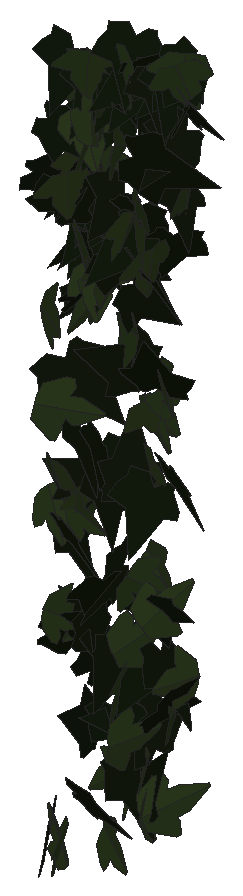
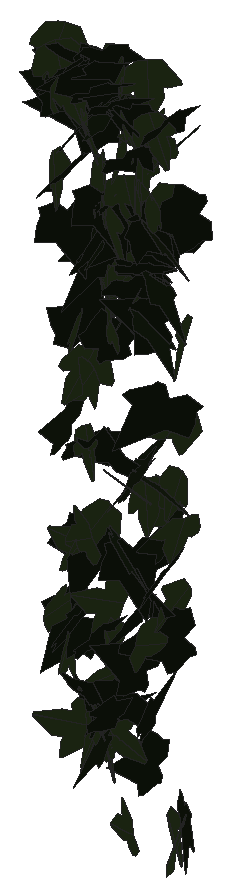
# SketchUp Ruby script. Lengths in inches.
U = 1.inch
M = Sketchup.active_model
def pt(a) = Geom::Point3d.new(a.map { |v| v * U })
def face(e, loops, mat)
  f = e.add_face(loops[0].map { |a| pt(a) })
  loops[1..].each { |l| e.add_face(l.map { |a| pt(a) }).erase! }
  f.material = f.back_material = mat if mat
  f
end
# faces: each face lists its corners as indices into pts; further lists are holes
def faces(e, pts, list, mat = nil) = list.each { |f| face(e, (f[0].is_a?(Array) ? f : [f]).map { |l| l.map { |i| pts[i] } }, mat) }
# xy, xz, yz: faces in a plane at the given z, y or x. An outline is a flat list of corners, or four numbers for a rectangle; further outlines are holes
def ring(l) = l.size == 4 ? [[l[0], l[1]], [l[2], l[1]], [l[2], l[3]], [l[0], l[3]]] : l.each_slice(2).to_a
def flat(e, list, mat, &to3) = list.each { |f| face(e, (f[0].is_a?(Array) ? f : [f]).map { |l| ring(l).map { |u, v| to3.(u, v) } }, mat) }
def xy(e, z, list, mat = nil) = flat(e, list, mat) { |x, y| [x, y, z] }
def xz(e, y, list, mat = nil) = flat(e, list, mat) { |x, z| [x, y, z] }
def yz(e, x, list, mat = nil) = flat(e, list, mat) { |y, z| [x, y, z] }
def lines(e, pts, list) = list.each { |a, b| e.add_line(pt(pts[a]), pt(pts[b])) }
# prism: a flat outline (further loops are holes) pulled along v
def prism(e, loops, v, mat = nil)
  f = face(e, loops, mat); d = Geom::Vector3d.new(v.map { |x| x * U })
  f.pushpull(f.normal.samedirection?(d) ? d.length : -d.length)
end
def box(e, o, s, mat = nil) = prism(e, [[o, [o[0] + s[0], o[1], o[2]], [o[0] + s[0], o[1] + s[1], o[2]], [o[0], o[1] + s[1], o[2]]]], [0, 0, s[2]], mat)
def at(x, y, z, deg = 0) = Geom::Transformation.translation(pt([x, y, z])) * Geom::Transformation.rotation(ORIGIN, Z_AXIS, deg.degrees)
def axes(o, x, y, z) = Geom::Transformation.new([*x, 0, *y, 0, *z, 0, *pt(o).to_a, 1])
def part(name) = M.definitions.add(name)
# library, detail: a bought-in or finely detailed component or shape, given as its bounding box
def library(name, o, s) = part(name).tap { |d| box(d.entities, o, s) }
def detail(e, o, s) = box(e.add_group.entities, o, s)
def put(e, d, t, mat = nil) = e.add_instance(d, t).tap { |i| i.material = mat if mat }
def group(e, t, mat = nil) = e.add_group.tap { |g| g.transformation = t; g.material = mat if mat }.entities
root = M.entities
M.materials.add("efeu1").color = [18, 25, 13]
M.materials.add("efeu2").color = [43, 57, 29]
c1 = part("ivyleaf_9")
p = [[1.54,2.16,1.25],[1.36,2.04,1.19],[-0.21,0.99,0.68],[-0.71,1.11,0.82],[-0.85,0.86,0.67],[-0.8,0.17,0.21],
  [-0.9,-0.01,0.1],[-0.67,-0.16,-0.02],[-0.08,-0.08,-0.05],[-0.03,-0.6,-0.4],[0.65,-0.88,-0.66],[0.83,-0.6,-0.49],
  [1.29,-0.42,-0.43],[1.8125,-0.07,-0.26],[1.21,0.44,0.15]]
faces(c1.entities,p,[[0,1,2,3,4,5,6,7,8,9,10,11,12,13,14]],"efeu1")
c2 = part("ivyleaf_10")
p = [[0,0.5,-0.03],[-0.0625,2.02,-0.43],[-0.19,2.01,-0.46],[-0.54,1.05,-0.29],[-0.52,0.625,-0.18],[-0.83,0.76,-0.28],
  [-1.16,0.64,-0.33],[-1.15,0.33,-0.24],[-0.77,-0.39,0.02],[-0.3,-0.51,0.16],[0.04,-0.48,0.23],[-0.02,2.01,-0.4375],
  [-0.06,2.01,-0.43],[0.04,-0.49,0.23],[0.67,-0.49,0.14],[1.38,0.36,-0.2],[1.375,0.51,-0.24],[0.81,0.65,-0.19],
  [0.62,0.59,-0.15],[0.6,1.09,-0.28],[0.5,1.23,-0.31]]
faces(c2.entities,p,[[0,1,2,3,4,5,6,7,8,9,10],[11,12,0,13,14,15,16,17,18,19,20]],"efeu2")
put(root,c1,axes([558.99,128.62,206.93],[-0.14033,0.02184,-1.08873],[-1.0012,0.42913,0.13765],[0.42827,1.01038,-0.03493]))
put(root,c2,axes([558.67,129.81,205.36],[-0.53555,0.90235,-0.1716],[-0.12374,0.12595,1.04848],[0.91014,0.54809,0.04157]))
put(root,c2,axes([558.25,129.72,221.42],[0.26299,0.95751,0.15924],[0.04787,0.15199,-0.99295],[-0.96948,0.26725,-0.00583]))
put(root,c2,axes([558.71,128.875,230.33],[-0.41315,0.69461,0.69183],[-0.42365,0.55054,-0.80575],[-0.8841,-0.58841,0.06281]))
put(root,c1,axes([557.92,129.1875,236.32],[0.17224,0.54015,-0.81604],[0.28185,0.76609,0.56658],[0.93715,-0.32968,-0.02042]))
put(root,c1,axes([558.34,130.9375,241.17],[-0.27235,-0.93235,0.29323],[-0.01478,-0.30044,-0.96899],[0.97726,-0.26437,0.06706]))
put(root,c1,axes([559.01,130.45,233.21],[-0.61672,0.77611,-0.04246],[0.03203,-0.02879,-0.99128],[-0.77661,-0.61751,-0.00716]))
put(root,c1,axes([558.23,130.81,219.78],[0.48249,-0.80704,-0.27],[-0.14212,0.2296,-0.94027],[0.83906,0.50297,-0.00401]))
put(root,c1,axes([559.04,130.875,235.99],[-0.8604,0.40877,-0.20405],[0.16752,-0.12253,-0.95181],[-0.42505,-0.87574,0.03792]))
put(root,c2,axes([559.12,130.72,240.85],[-0.85129,-0.027,0.49047],[-0.47595,-0.19735,-0.83696],[0.12148,-0.96245,0.15786]))
put(root,c1,axes([559.45,130.33,230.87],[-0.35302,0.84005,0.36834],[-0.31546,0.25941,-0.89396],[-0.8613,-0.43932,0.17645]))
put(root,c2,axes([558.89,129.25,223.13],[-0.86155,0.40048,-0.04378],[0.0411,-0.01544,-0.95007],[-0.40077,-0.86252,-0.00332]))
put(root,c2,axes([559.09,130.33,236.95],[0.01574,-0.90176,0.44705],[0.02742,-0.44655,-0.90173],[1.00612,0.02628,0.01758]))
put(root,c1,axes([559.12,131.28,236.4375],[-0.30759,0.37254,-0.86401],[0.44342,-0.74434,-0.4788],[-0.82987,-0.53581,0.06441]))
put(root,c2,axes([559.0625,129.375,206.56],[0.48481,-0.8241,0.02003],[0.01483,-0.01451,-0.95611],[0.82421,0.485,0.00543]))
put(root,c1,axes([559.8,129.625,222.84],[-0.36512,0.6723,0.51093],[-0.54966,0.23334,-0.69984],[-0.64102,-0.58302,0.30907]))
put(root,c1,axes([558.51,129.7,234.65],[-0.08443,-0.16044,0.99072],[1.00342,0.00694,0.08663],[-0.02063,0.99429,0.15926]))
put(root,c2,axes([559.21,131.25,216.0625],[0.0966,0.37472,-0.88999],[-0.25262,-0.85347,-0.38677],[-0.93203,0.27016,0.01259]))
put(root,c2,axes([559.29,129.4375,236.31],[-0.49063,-0.8754,-0.07136],[0.02747,0.0664,-1.00348],[0.87788,-0.49133,-0.00848]))
put(root,c1,axes([558.64,130.23,227.54],[-0.08979,-0.46984,-1.10499],[0.35695,1.04754,-0.47442],[1.14645,-0.36295,0.06117]))
put(root,c2,axes([558.62,129.08,226.04],[-0.13884,-0.24942,-1.05061],[0.96555,0.44555,-0.23337],[0.48342,-0.96153,0.16439]))
put(root,c2,axes([559.32,128.4375,217.12],[-0.04611,0.53566,0.801],[-0.13304,0.7907,-0.53643],[-0.95438,-0.13611,0.03608]))
put(root,c1,axes([558.7,129.22,215.64],[0.6801,0.26796,0.73486],[0.68349,0.26993,-0.73098],[-0.38035,0.96421,0.00042]))
put(root,c1,axes([559.4375,131.46,234.24],[-0.78252,-0.61482,0.02829],[0.13153,-0.21175,-0.96385],[0.60126,-0.75386,0.24766]))
put(root,c1,axes([559,128.67,239.25],[0.70392,-0.50862,-0.52755],[-0.16527,0.60247,-0.80138],[0.71392,0.64097,0.33463]))
put(root,c1,axes([559.65,131.09,234.16],[-0.79091,-0.55455,-0.11469],[0.09217,0.06832,-0.96595],[0.55873,-0.79626,-0.003]))
put(root,c1,axes([559.08,129.39,220.6],[0.6914,-0.5788,0.15277],[0.11818,-0.09683,-0.90169],[0.58684,0.70143,0.00159]))
put(root,c1,axes([559.45,130.46,233.45],[0.66187,-0.53962,-0.55674],[-0.40225,0.3868,-0.85311],[0.66284,0.77357,0.03821]))
put(root,c1,axes([559.34,129.76,230.8],[0.18284,0.92021,-0.39849],[0.0771,0.39095,0.9382],[0.99982,-0.19843,0.00052]))
put(root,c1,axes([559.89,130.1875,211.32],[-0.15828,0.0297,0.95286],[-0.32432,-0.90997,-0.02551],[0.89646,-0.32396,0.15901]))
put(root,c1,axes([559.4375,130.16,224.61],[0.3603,-0.90096,0.33872],[0.12813,-0.31356,-0.97033],[0.95396,0.3824,0.0024]))
put(root,c2,axes([559.66,130.98,237.56],[0.55503,-0.64106,0.48861],[0.48472,-0.20853,-0.8242],[0.644,0.70944,0.19925]))
put(root,c2,axes([560.16,129.75,222.45],[-0.21734,-0.92722,-0.07315],[0.01697,0.07115,-0.95235],[0.92994,-0.218,0.00029]))
put(root,c2,axes([560.17,129.84,238.41],[0.20873,-0.88624,-0.43695],[-0.01941,0.44282,-0.90744],[0.98791,0.19595,0.07449]))
put(root,c1,axes([560.08,131.25,239.17],[-0.53453,-0.8444,0.10638],[0.01515,-0.13504,-0.99579],[0.85094,-0.52802,0.08455]))
put(root,c1,axes([559.67,131.15,223.6],[0.08003,-0.70565,0.66439],[0.17582,-0.64502,-0.70626],[0.95312,0.17823,0.07449]))
put(root,c1,axes([559.99,131.03,233.08],[-0.4486,-0.83389,-0.21901],[0.16097,0.16153,-0.94476],[0.84701,-0.47235,0.06355]))
put(root,c1,axes([560.3,130.47,241],[-0.84195,-0.49876,-0.15488],[0.1388,0.06956,-0.97853],[0.50347,-0.85325,0.01076]))
put(root,c2,axes([560.45,129.35,242.29],[-0.78359,-0.66818,0.08016],[-0.06965,-0.04185,-1.02971],[0.66936,-0.78657,-0.01331]))
put(root,c2,axes([560.57,130.64,237.3125],[-0.9298,-0.1154,0.30767],[-0.27239,-0.24579,-0.91537],[0.1838,-0.94804,0.19987]))
put(root,c2,axes([560.21,130.14,231.15],[-0.0111,-0.40165,0.90513],[0.21172,-0.88521,-0.39022],[0.96734,0.18913,0.09579]))
put(root,c1,axes([561,128.95,216.64],[-0.25972,0.29871,0.94969],[-0.61467,0.72396,-0.39581],[-0.78315,-0.66727,-0.0043]))
put(root,c2,axes([560.19,129.03,234.25],[-0.68525,0.6821,-0.13138],[0.08987,-0.09595,-0.96685],[-0.6888,-0.6911,0.00456]))
put(root,c1,axes([560.36,131.3,223.51],[-0.8108,-0.24209,-0.34921],[0.40316,-0.20065,-0.79697],[0.13422,-0.8597,0.28434]))
put(root,c2,axes([560.52,129.26,239.06],[-0.09308,0.93086,-0.54961],[-0.1256,0.5386,0.93348],[1.07369,0.1437,0.06155]))
put(root,c1,axes([559.98,130.14,214.08],[0.13359,-0.11991,1.05032],[0.78522,0.72009,-0.01766],[-0.70781,0.77621,0.17864]))
put(root,c1,axes([560.91,130.75,240.5],[-0.97074,0.21539,0.07325],[-0.07451,0.00233,-0.99426],[-0.21496,-0.9735,0.01383]))
put(root,c2,axes([560,129.45,239.27],[0.7958,0.55612,0.33148],[0.2758,0.184,-0.97084],[-0.58573,0.84221,-0.00678]))
put(root,c2,axes([559.75,129.22,221.58],[0.07631,-0.1076,0.90905],[0.91477,0.04286,-0.07172],[-0.03402,0.91124,0.11071]))
put(root,c2,axes([560.35,129.73,232.33],[0.63947,0.7254,0.09194],[0.05587,0.07331,-0.96699],[-0.72906,0.64187,0.00654]))
put(root,c1,axes([560.23,129.01,208.86],[0.73504,-0.38675,0.48989],[0.44125,-0.21331,-0.83045],[0.44144,0.85719,0.01437]))
put(root,c2,axes([560.27,130.65,206.31],[0.27672,-0.04353,0.97521],[0.94609,-0.23776,-0.27907],[0.24049,0.98543,-0.02426]))
put(root,c2,axes([560.99,130.02,240.53],[0.37829,-0.89853,0.15926],[0.08484,-0.13702,-0.9746],[0.90858,0.3869,0.0247]))
put(root,c1,axes([561.27,129.21,218.86],[0.16936,0.88596,-0.48783],[-0.0822,-0.48093,-0.90196],[-1.00804,0.18806,-0.00841]))
put(root,c2,axes([561.19,129.99,232.85],[-0.1984,-0.95037,0.21572],[-0.02604,-0.21489,-0.97069],[0.9742,-0.19929,0.01799]))
put(root,c1,axes([560.66,130.15,222.73],[0.21157,-0.965,0.20893],[0.04249,-0.20457,-0.98792],[0.98644,0.21579,-0.00226]))
put(root,c1,axes([561.09,130.97,241.22],[-0.61139,-0.7967,0.11583],[0.11322,-0.22909,-0.97808],[0.79708,-0.57855,0.22778]))
put(root,c1,axes([561.45,131.3,211.76],[-0.05574,-0.69209,-0.58924],[-0.01887,-0.58934,0.69399],[-0.90875,0.05469,0.02173]))
put(root,c1,axes([561.7,129.79,219.45],[-0.92418,0.45294,-0.32855],[0.29713,-0.14028,-1.0292],[-0.47415,-0.97076,-0.00457]))
put(root,c2,axes([561.97,129.93,210.24],[-0.43773,-0.25611,0.80676],[-0.6712,-0.44833,-0.5065],[0.5157,-0.80091,0.02555]))
put(root,c2,axes([561.59,129.53,238.75],[0.25822,-0.48953,-0.86004],[-0.14162,0.86141,-0.53283],[0.97941,0.25362,0.1497]))
put(root,c1,axes([560.94,130.25,212.52],[-0.29374,-0.31991,-0.87643],[0.63983,0.59967,-0.43333],[0.67904,-0.70343,0.02918]))
put(root,c1,axes([561.24,129.99,215.45],[-0.0653,-0.97947,0.57005],[-0.04544,-0.56827,-0.98162],[1.13236,-0.07928,-0.00652]))
put(root,c1,axes([561.54,130.09,236.18],[-0.34519,-0.75817,0.56128],[-0.07354,-0.57423,-0.82089],[0.94045,-0.32319,0.14183]))
put(root,c2,axes([562.1,129.94,234.91],[0.66039,-0.42115,-0.66754],[-0.50251,0.44685,-0.77904],[0.60866,0.82587,0.0811]))
put(root,c1,axes([562.1,129.88,223.26],[-1.05025,0.14244,0.21134],[0.20818,-0.03756,1.05982],[0.14703,1.07064,0.00906]))
put(root,c2,axes([561.79,130,214.72],[0.52408,-1.03025,0.2683],[0.11556,-0.24223,-1.15587],[1.05832,0.53663,-0.00665]))
put(root,c2,axes([561.64,129.81,242.56],[-0.68138,0.48042,-0.54987],[0.33141,-0.46669,-0.81842],[-0.65063,-0.74084,0.15898]))
put(root,c1,axes([561.7,130.51,210.33],[0.78926,-0.39965,-0.35194],[-0.30862,0.16952,-0.88461],[0.43397,0.84738,0.01098]))
put(root,c1,axes([562.08,131,241.52],[-0.63703,-0.7684,0.18306],[0.03067,-0.25906,-0.98067],[0.78931,-0.61008,0.18585]))
put(root,c1,axes([562.375,129.86,235.9],[0.4044,0.54385,-0.7747],[-0.42202,-0.65047,-0.67694],[-0.84725,0.58359,-0.03258]))
put(root,c1,axes([562.49,129.83,228.67],[-0.04315,-0.05191,1.03692],[-0.90311,-0.51007,-0.06312],[0.51214,-0.90382,-0.02394]))
put(root,c1,axes([562.47,130.64,242.0625],[-0.77811,-0.5283,0.39865],[-0.32311,-0.23376,-0.94044],[0.5776,-0.84245,0.01096]))
put(root,c1,axes([561.94,130.4,243.27],[-0.54641,-0.77859,-0.31056],[0.2449,0.20626,-0.948],[0.80167,-0.59369,0.07792]))
put(root,c1,axes([561.5,130.54,240.37],[0.41774,-0.85171,0.28529],[0.31362,-0.15653,-0.92652],[0.84169,0.48103,0.20364]))
put(root,c2,axes([562.21,129.98,209.88],[0.58641,-0.77525,-0.09309],[-0.05635,0.07411,-0.97206],[0.77879,0.58911,-0.00023]))
put(root,c1,axes([561.89,128.97,234.13],[0.07976,-0.092,-1.02629],[-0.06477,1.02688,-0.09708],[1.02837,0.07181,0.07348]))
put(root,c2,axes([561.72,130.14,230.07],[0.56125,-0.3845,0.69192],[0.6574,-0.24606,-0.66998],[0.44093,0.85628,0.11817]))
put(root,c1,axes([562.29,130.75,214.96],[-0.29919,-0.83094,0.40734],[-0.11496,-0.39141,-0.88288],[0.91824,-0.31975,0.02219]))
put(root,c2,axes([563.02,128.8,230.99],[0.16737,-0.23559,-1.0808],[-0.69784,0.82565,-0.28804],[0.85829,0.71725,-0.02344]))
put(root,c1,axes([562.72,129.57,235],[-0.72792,-0.62121,0.29921],[-0.21163,-0.2128,-0.95667],[0.65623,-0.7577,0.02338]))
put(root,c2,axes([562.46,129.27,235.59],[0.15148,-0.92723,0.34655],[0.13361,-0.32822,-0.9366],[0.98081,0.18791,0.07406]))
put(root,c2,axes([562.17,129.37,216.21],[0.20845,0.31534,-0.9882],[0.6122,0.77628,0.37685],[0.83737,-0.64604,-0.02953]))
put(root,c2,axes([563.08,129.21,236.82],[-0.61335,0.39923,0.74009],[-0.67475,0.31301,-0.72805],[-0.50183,-0.90883,0.07436]))
put(root,c1,axes([563.14,130.14,211.68],[-1.06679,0.20701,-0.21356],[-0.21057,0.0359,1.08668],[0.21004,1.08736,0.00478]))
put(root,c2,axes([563.02,130.24,224.29],[-0.70586,0.30113,0.51014],[-0.5129,0.08637,-0.76067],[-0.29639,-0.86661,0.10145]))
put(root,c2,axes([562.49,130.82,239.59],[0.71658,-0.64273,0.24249],[0.16228,-0.18211,-0.96223],[0.66751,0.73425,-0.02639]))
put(root,c1,axes([562.14,130.04,241.74],[0.59621,0.23261,0.76126],[0.68152,0.34226,-0.63834],[-0.41128,0.90435,0.04578]))
put(root,c2,axes([562.54,128.53,212.33],[-0.04399,-0.05123,-1.07154],[0.46708,0.96454,-0.06528],[0.96575,-0.46883,-0.01723]))
put(root,c2,axes([562.9,129.67,210.95],[0.65049,-0.76511,-0.13929],[-0.08862,0.10748,-1.00426],[0.77262,0.6565,0.00208]))
put(root,c1,axes([562.4375,129.16,210.9],[0.41602,-0.94136,-0.35014],[-0.12257,0.32858,-1.029],[0.99686,0.43326,0.01961]))
put(root,c1,axes([562.83,129.29,232.84],[0.29116,-0.37408,-0.94032],[-0.39938,0.85657,-0.46442],[0.92986,0.48504,0.09496]))
put(root,c1,axes([562.58,131.05,239.79],[0.39403,-0.92841,-0.05768],[0.01367,0.06842,-1.0078],[0.9301,0.39231,0.03925]))
put(root,c2,axes([563.33,131.11,241.52],[-0.24789,-0.91344,0.329],[0.0212,-0.34457,-0.94068],[0.97065,-0.22575,0.10457]))
put(root,c2,axes([563.64,128.99,209.1875],[-0.10796,0.14861,1.08255],[-0.67583,0.84572,-0.1835],[-0.85864,-0.68435,0.00832]))
put(root,c2,axes([563.67,128.55,234.88],[-0.1,0.19695,-1.11766],[-0.40322,1.04262,0.21981],[1.06083,0.41486,-0.02181]))
put(root,c1,axes([562.95,129.36,209.36],[-0.4095,0.55901,0.83051],[0.43162,-0.71104,0.69141],[0.9033,0.59318,0.04612]))
put(root,c2,axes([563.14,128.84,219.82],[-0.2753,-0.6108,-0.79172],[0.40807,0.68106,-0.66732],[0.91289,-0.48864,0.05954]))
put(root,c2,axes([562.59,130.58,219.66],[0.49056,-0.06759,0.9252],[0.92061,-0.09337,-0.49495],[0.1142,1.04304,0.01565]))
put(root,c1,axes([562.71,129.68,233.76],[0.81253,-0.63803,0.13642],[0.10721,-0.08435,-1.0331],[0.64359,0.81957,-0.00013]))
put(root,c2,axes([563.05,130.07,227.14],[-0.7628,0.29015,-0.52841],[0.43074,-0.33387,-0.80514],[-0.42174,-0.8658,0.1334]))
put(root,c1,axes([563.42,129.64,223.61],[-0.46835,-0.89364,0.00731],[-0.00122,-0.00761,-1.00893],[0.89367,-0.46835,0.00246]))
put(root,c1,axes([563.25,130.59,242.05],[-0.24911,-0.94187,-0.24289],[0.09663,0.22553,-0.97363],[0.96787,-0.26493,0.03469]))
put(root,c1,axes([563.79,130.48,234.85],[0.28653,0.70685,-0.6284],[-0.19726,-0.5975,-0.76204],[-0.92499,0.34637,-0.03215]))
put(root,c2,axes([563.42,129.49,227.49],[-0.54023,-0.6968,-0.55772],[0.37065,0.41791,-0.88114],[0.81191,-0.65442,0.03116]))
put(root,c2,axes([563.72,129.12,234.55],[-0.16513,-1.04166,-0.11128],[0.01649,0.11006,-1.05467],[1.04746,-0.16595,-0.00094]))
put(root,c1,axes([563.6,129.1,218.82],[0.85669,0.54437,-0.40831],[-0.35372,-0.20457,-1.01489],[-0.58132,0.9267,0.01581]))
put(root,c1,axes([563.22,130.51,215.66],[0.48561,-0.94616,-0.30487],[-0.14226,0.26967,-1.0635],[0.98384,0.50601,-0.0033]))
put(root,c1,axes([563.54,131.08,241.94],[-0.20221,-0.98144,0.1434],[0.01138,-0.14864,-1.00123],[0.9918,-0.19839,0.04073]))
put(root,c2,axes([564.05,130.87,242.69],[-0.67668,-0.7453,0.17455],[-0.03801,-0.19997,-1.0012],[0.76453,-0.66961,0.10472]))
put(root,c1,axes([564.28,130.68,241.02],[-0.76836,0.60828,-0.2117],[0.18019,-0.11336,-0.97973],[-0.61835,-0.78888,-0.02244]))
put(root,c1,axes([564.35,130.87,242.57],[-0.97826,-0.27368,0.10726],[-0.10349,-0.0282,-1.01583],[0.27513,-0.98372,-0.00072]))
put(root,c1,axes([563.8,129.42,228.5625],[0.9547,-0.03705,0.46223],[-0.46202,0.01426,0.95541],[-0.03956,-1.06061,-0.0033]))
put(root,c2,axes([564.29,129.69,213.69],[0.03494,-0.21739,-1.01749],[-0.23292,0.9906,-0.21964],[1.01405,0.23502,-0.01539]))
put(root,c2,axes([564.08,129.48,229.1],[-0.48174,0.80136,0.12608],[-0.08158,0.09804,-0.93482],[-0.8071,-0.48822,0.01923]))
put(root,c1,axes([563.6875,130.94,237.04],[0.17924,-0.96788,0.04189],[0.05997,-0.03144,-0.9829],[0.96693,0.18137,0.05319]))
put(root,c2,axes([563.82,129.05,218.22],[0.39459,0.42653,-0.89712],[0.61697,0.65131,0.58103],[0.77852,-0.73234,-0.00577]))
put(root,c2,axes([564.32,130.65,237.17],[0.30423,-0.93063,-0.1595],[0.05916,0.18603,-0.97261],[0.94235,0.28877,0.11255]))
put(root,c1,axes([564.46,128.82,214.36],[0.32634,0.88829,0.60233],[0.20699,0.56565,-0.94634],[-1.05309,0.38645,0.00065]))
put(root,c1,axes([563.48,128.61,239.16],[0.48056,0.17396,-1.14382],[0.81944,0.82318,0.46947],[0.81675,-0.92824,0.20198]))
put(root,c1,axes([564.8125,129.89,240.23],[-0.95354,-0.27346,-0.08998],[0.09739,-0.01344,-0.99119],[0.27091,-0.95768,0.03961]))
put(root,c2,axes([563.97,129.1,209.51],[0.25689,0.25622,-1.09402],[0.85497,0.68361,0.36087],[0.72908,-0.89193,-0.0377]))
put(root,c1,axes([563.99,130.1,224.43],[0.61047,-0.68748,0.3372],[0.21303,-0.26174,-0.9193],[0.7355,0.64643,-0.01361]))
put(root,c1,axes([563.82,130.8,240.97],[0.55309,-0.49712,0.70228],[0.54878,-0.4392,-0.74309],[0.6627,0.77859,0.02922]))
put(root,c2,axes([564.67,130.31,215.1875],[-0.18526,0.1902,0.96966],[0.1468,-0.97031,0.21838],[0.97717,0.18183,0.15103]))
put(root,c2,axes([564.67,129.84,242.92],[-0.73672,-0.62403,-0.29686],[0.2307,0.18693,-0.96547],[0.6514,-0.77197,0.00619]))
